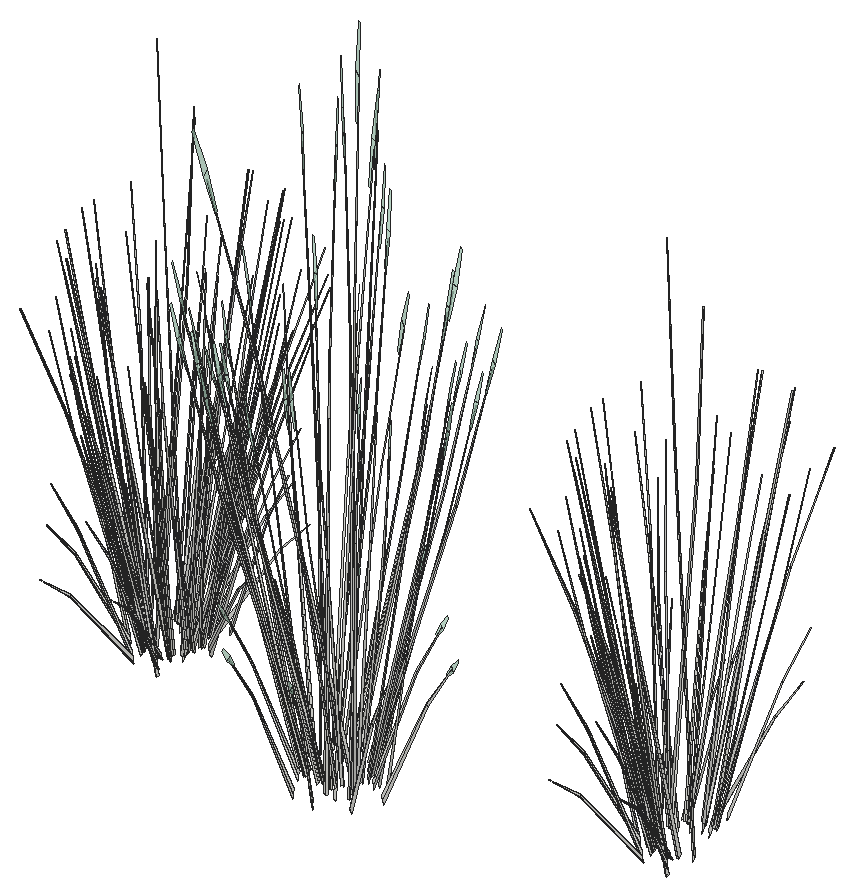
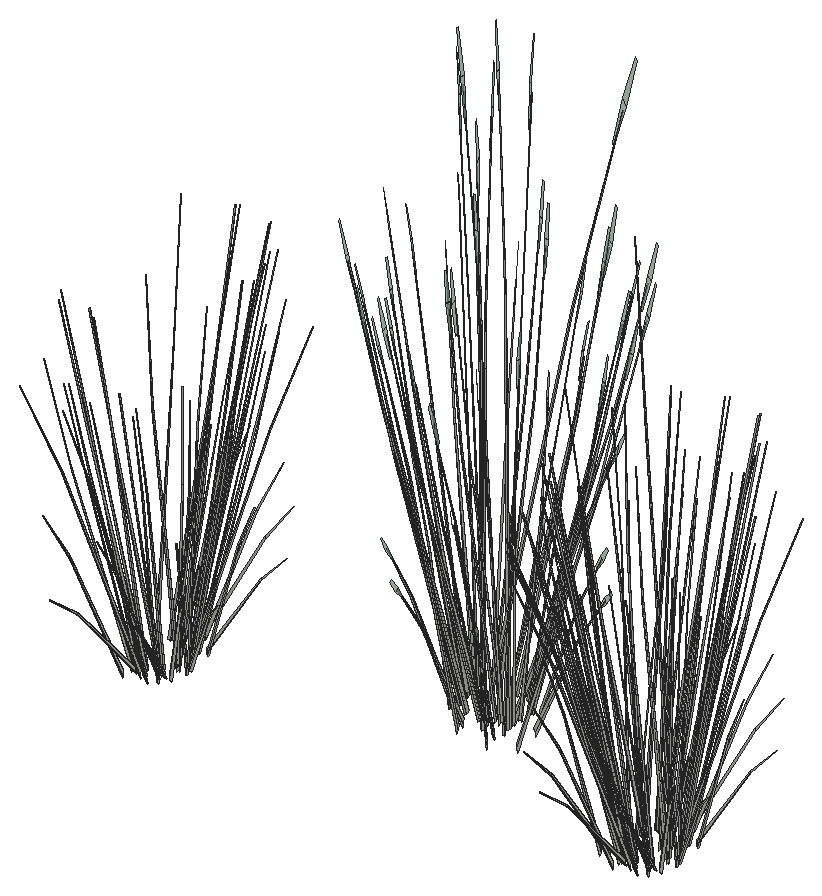
# SketchUp Ruby script. Lengths in inches.
U = 1.inch
M = Sketchup.active_model
def pt(a) = Geom::Point3d.new(a.map { |v| v * U })
def face(e, loops, mat)
  f = e.add_face(loops[0].map { |a| pt(a) })
  loops[1..].each { |l| e.add_face(l.map { |a| pt(a) }).erase! }
  f.material = f.back_material = mat if mat
  f
end
# faces: each face lists its corners as indices into pts; further lists are holes
def faces(e, pts, list, mat = nil) = list.each { |f| face(e, (f[0].is_a?(Array) ? f : [f]).map { |l| l.map { |i| pts[i] } }, mat) }
# xy, xz, yz: faces in a plane at the given z, y or x. An outline is a flat list of corners, or four numbers for a rectangle; further outlines are holes
def ring(l) = l.size == 4 ? [[l[0], l[1]], [l[2], l[1]], [l[2], l[3]], [l[0], l[3]]] : l.each_slice(2).to_a
def flat(e, list, mat, &to3) = list.each { |f| face(e, (f[0].is_a?(Array) ? f : [f]).map { |l| ring(l).map { |u, v| to3.(u, v) } }, mat) }
def xy(e, z, list, mat = nil) = flat(e, list, mat) { |x, y| [x, y, z] }
def xz(e, y, list, mat = nil) = flat(e, list, mat) { |x, z| [x, y, z] }
def yz(e, x, list, mat = nil) = flat(e, list, mat) { |y, z| [x, y, z] }
def lines(e, pts, list) = list.each { |a, b| e.add_line(pt(pts[a]), pt(pts[b])) }
# prism: a flat outline (further loops are holes) pulled along v
def prism(e, loops, v, mat = nil)
  f = face(e, loops, mat); d = Geom::Vector3d.new(v.map { |x| x * U })
  f.pushpull(f.normal.samedirection?(d) ? d.length : -d.length)
end
def box(e, o, s, mat = nil) = prism(e, [[o, [o[0] + s[0], o[1], o[2]], [o[0] + s[0], o[1] + s[1], o[2]], [o[0], o[1] + s[1], o[2]]]], [0, 0, s[2]], mat)
def at(x, y, z, deg = 0) = Geom::Transformation.translation(pt([x, y, z])) * Geom::Transformation.rotation(ORIGIN, Z_AXIS, deg.degrees)
def axes(o, x, y, z) = Geom::Transformation.new([*x, 0, *y, 0, *z, 0, *pt(o).to_a, 1])
def part(name) = M.definitions.add(name)
# library, detail: a bought-in or finely detailed component or shape, given as its bounding box
def library(name, o, s) = part(name).tap { |d| box(d.entities, o, s) }
def detail(e, o, s) = box(e.add_group.entities, o, s)
def put(e, d, t, mat = nil) = e.add_instance(d, t).tap { |i| i.material = mat if mat }
def group(e, t, mat = nil) = e.add_group.tap { |g| g.transformation = t; g.material = mat if mat }.entities
root = M.entities
M.materials.add("LightPink_Translucent").color = [175, 214, 192]
M.materials["LightPink_Translucent"].alpha = 0.75
c1 = part("blade")
p = [[2.15,0.21,22],[0,0.17,0],[0.09,0.45,0],[2.18,0.31,22],[2.29,0.31,22],[0.38,0.45,0],
  [2.48,0.24,33],[2.49,0.24,33],[2.48,0.22,33]]
faces(c1.entities,p,[[0,1,2,3],[4,5,2,3],[6,3,4,7],[8,0,3,6]])
c2 = part("blade with seeds\#1")
put(c2.entities,c1,at(0,0,0))
c3 = part("seeds")
p = [[0.3,-0.1,1.38],[-0.01,-0.03,1.59],[-0.01,-0.03,0.03],[0.14,-0.07,-0.07],[0.29,-0.03,3],[0.15,0.01,3.11]]
faces(c3.entities,p,[[0,1,2,3],[1,0,4,5]],"LightPink_Translucent")
c4 = part("blade with seeds")
put(c4.entities,c1,at(0,0,0))
put(c4.entities,c3,axes([2.4,0.25,30.99],[1.5799,-0.05474,1.17369],[-0.12525,1.92788,0.29478],[-0.07173,-0.02425,1.56792]))
put(root,c2,axes([371.53,244.35,139.9],[0.12234,-0.11364,1.40588],[0.103,0.52511,0.11368],[-0.19206,0.11868,0.601]))
put(root,c2,axes([370.72,243.48,140.59],[-0.05342,0.07604,1.43516],[0.03387,0.50744,-0.22697],[-0.12778,0.08099,0.1151]))
put(root,c2,axes([371.1,241.31,140.58],[0.0291,0.05049,1.45516],[-0.09819,0.49465,-0.1375],[-0.12701,0.01791,0.25751]))
put(root,c2,axes([371.375,241.2,140.59],[-0.07584,0.0048,1.43516],[-0.21918,0.40531,-0.22697],[-0.13286,-0.06266,0.1151]))
put(root,c2,axes([371.75,242.57,139.9],[0.13097,0.09256,1.40588],[-0.27104,0.38832,0.11368],[-0.16893,-0.17518,0.601]))
put(root,c2,axes([371.36,242.9,140.43],[-0.29303,-0.14987,-0.29052],[0.08547,-0.43725,0.37506],[-0.11798,0.04009,0.71765]))
put(root,c2,axes([370.54,244,140.58],[0.04567,0.00927,1.45516],[0.16576,0.45742,-0.1375],[-0.08473,0.1346,0.25751]))
put(root,c2,axes([371.54,242.71,140.85],[0.17741,0.48648,-0.09976],[-0.31487,0.23906,-0.55369],[-0.13269,0.06419,0.84132]))
put(root,c2,axes([371.43,242.85,140.6],[0.09962,-0.48986,0.39379],[0.3275,0.16751,0.3247],[-0.12879,0.02944,0.81485]))
put(root,c2,axes([371.94,241.7,140.85],[-0.01888,0.54637,-0.09976],[-0.35746,-0.01493,-0.55369],[-0.13767,-0.03795,0.84132]))
put(root,c2,axes([371.4,242.72,140.6],[-0.1295,-0.36632,0.05275],[0.23615,-0.1793,0.41527],[-0.1041,0.03538,0.63322]))
put(root,c2,axes([371.47,244.16,140.43],[-0.30692,0.07678,-0.29052],[-0.08104,-0.43892,0.37506],[-0.08795,0.11789,0.71765]))
put(root,c2,axes([371.71,241.73,140.43],[-0.20062,-0.33637,-0.29052],[0.22908,-0.31842,0.37506],[-0.11639,-0.04845,0.71765]))
put(root,c2,axes([371.4375,243.97,140.6],[-0.24206,-0.22594,0.05275],[0.14093,-0.32175,0.41527],[-0.07761,0.10402,0.63322]))
put(root,c2,axes([371.91,245.11,139.9],[0.06565,-0.18466,1.40588],[0.27542,0.38215,0.11368],[-0.12424,0.23818,0.601]))
put(root,c2,axes([371.41,243.87,141.17],[0.3653,0.33178,-0.11173],[-0.21045,0.48049,-0.62013],[-0.10321,0.16702,0.94228]))
put(root,c2,axes([371.79,241.74,140.6],[0.25999,-0.354,0.39379],[0.22422,0.37594,0.3247],[-0.12198,-0.0653,0.81485]))
put(root,c2,axes([371.81,241.61,140.6],[0.01775,-0.40853,0.05275],[0.2681,0.0112,0.41527],[-0.1027,-0.04275,0.63322]))
put(root,c2,axes([371.31,245.14,140.59],[-0.00269,0.10696,1.43516],[0.26896,0.34054,-0.22697],[-0.05496,0.1817,0.1151]))
put(root,c2,axes([372.65,241.1,140.85],[-0.21011,0.45986,-0.09976],[-0.30427,-0.26493,-0.55369],[-0.10577,-0.12992,0.84132]))
put(root,c2,axes([372.55,239.97,140.58],[-0.00289,0.06493,1.45516],[-0.31009,0.26964,-0.1375],[-0.10196,-0.10828,0.25751]))
put(root,c2,axes([373.79,243,139.45],[0.15365,-0.4296,1.24087],[0.33102,0.42086,0.4907],[-0.19619,0.18851,1.04025]))
put(root,c2,axes([371.91,245.03,140.6],[-0.28975,-0.02503,0.05275],[0.00794,-0.378,0.41527],[-0.03032,0.1448,0.63322]))
put(root,c2,axes([372.01,245.18,140.43],[-0.23857,0.28286,-0.29052],[-0.22584,-0.32298,0.37506],[-0.03436,0.1641,0.71765]))
put(root,c2,axes([372.43,240.97,140.43],[-0.05446,-0.43273,-0.29052],[0.31131,-0.11427,0.37506],[-0.08362,-0.12401,0.71765]))
put(root,c2,axes([372.5,241.03,140.6],[0.35069,-0.12329,0.39379],[0.06086,0.48364,0.3247],[-0.08248,-0.14254,0.81485]))
put(root,c2,axes([372.57,240.93,140.6],[0.16025,-0.34128,0.05275],[0.22821,0.1987,0.41527],[-0.07378,-0.10942,0.63322]))
put(root,c2,axes([372.92,239.73,140.59],[-0.05804,-0.06898,1.43516],[-0.35603,0.0883,-0.22697],[-0.0675,-0.17309,0.1151]))
put(root,c2,axes([371.53,245.55,140.58],[0.03803,-0.03685,1.45516],[0.34183,0.17767,-0.1375],[0.00247,0.17994,0.25751]))
put(root,c2,axes([371.98,244.86,140.85],[0.38751,0.02662,-0.09976],[-0.01059,0.50399,-0.55369],[-0.02692,0.19411,0.84132]))
put(root,c2,axes([373.47,241.08,140.85],[-0.34504,0.25013,-0.09976],[-0.16956,-0.44394,-0.55369],[-0.04552,-0.18708,0.84132]))
put(root,c2,axes([372.51,245.5,139.9],[-0.00863,-0.2062,1.40588],[0.37404,0.13679,0.11368],[-0.02314,0.29386,0.601]))
put(root,c2,axes([372.79,245.58,140.6],[-0.34743,-0.14045,0.39379],[0.1188,-0.46175,0.3247],[0.02088,0.18159,0.81485]))
put(root,c2,axes([372.7,245.62,140.6],[-0.25981,0.18259,0.05275],[-0.12717,-0.33295,0.41527],[0.02509,0.14677,0.63322]))
put(root,c2,axes([372.83,245.68,140.43],[-0.1063,0.41315,-0.29052],[-0.31012,-0.1205,0.37506],[0.02844,0.16634,0.71765]))
put(root,c2,axes([373.33,240.82,140.43],[0.1063,-0.41315,-0.29052],[0.31012,0.1205,0.37506],[-0.02844,-0.16634,0.71765]))
put(root,c2,axes([372.94,241.95,139.9],[0.00863,0.2062,1.40588],[-0.37404,-0.13679,0.11368],[0.02314,-0.29386,0.601]))
put(root,c2,axes([373.46,240.88,140.6],[0.25981,-0.18259,0.05275],[0.12717,0.33295,0.41527],[-0.02509,-0.14677,0.63322]))
put(root,c2,axes([373.37,240.92,140.6],[0.34743,0.14045,0.39379],[-0.1188,0.46175,0.3247],[-0.02088,-0.18159,0.81485]))
put(root,c2,axes([372.69,245.42,140.85],[0.34504,-0.25013,-0.09976],[0.16956,0.44394,-0.55369],[0.04552,0.18708,0.84132]))
put(root,c2,axes([374.49,240.09,140.58],[-0.03336,0.04495,1.45516],[-0.35758,-0.09833,-0.1375],[-0.02285,-0.17707,0.25751]))
put(root,c2,axes([373.04,245.9375,140.59],[0.04947,0.08118,1.43516],[0.36146,-0.00691,-0.22697],[0.04701,0.18608,0.1151]))
put(root,c2,axes([374.19,240.48,139.94],[-0.32031,0.09515,-0.02864],[-0.07364,-0.44972,-0.12987],[0.02031,-0.09391,0.42837]))
put(root,c2,axes([374.18,241.65,140.85],[-0.38751,-0.02662,-0.09976],[0.01059,-0.50399,-0.55369],[0.02692,-0.19411,0.84132]))
put(root,c2,axes([373.95,241.21,140.59],[-0.00644,-0.10664,1.43516],[-0.29603,-0.29251,-0.22697],[0.03908,-0.18969,0.1151]))
put(root,c2,axes([373.59,245.57,140.6],[-0.16025,0.34128,0.05275],[-0.22821,-0.1987,0.41527],[0.07378,0.10942,0.63322]))
put(root,c2,axes([373.66,245.47,140.6],[-0.35069,0.12329,0.39379],[-0.06086,-0.48364,0.3247],[0.08248,0.14254,0.81485]))
put(root,c2,axes([373.17,245.41,139.9],[-0.0806,-0.17249,1.40588],[0.37244,-0.14522,0.11368],[0.08417,0.2708,0.601]))
put(root,c2,axes([373.4,246.84,140.58],[0.01022,-0.06344,1.45516],[0.33667,-0.19627,-0.1375],[0.08837,0.12987,0.25751]))
put(root,c2,axes([373.73,245.53,140.43],[0.05446,0.43273,-0.29052],[-0.31131,0.11427,0.37506],[0.08362,0.12401,0.71765]))
put(root,c2,axes([374.16,241.32,140.43],[0.23857,-0.28286,-0.29052],[0.22584,0.32298,0.37506],[0.03436,-0.1641,0.71765]))
put(root,c2,axes([374.25,241.47,140.6],[0.28975,0.02503,0.05275],[-0.00794,0.378,0.41527],[0.03032,-0.1448,0.63322]))
put(root,c2,axes([374.15,241.43,140.6],[0.25108,0.36656,0.39379],[-0.26664,0.31614,0.3247],[0.04631,-0.17198,0.81485]))
put(root,c2,axes([372.68,242.3,140.39],[-0.19798,0.42958,1.1344],[-0.30825,-0.45359,0.48946],[0.18577,-0.1386,1.09651]))
put(root,c2,axes([373.54,242.34,139.9],[-0.06565,0.18466,1.40588],[-0.27542,-0.38215,0.11368],[0.12424,-0.23818,0.601]))
put(root,c2,axes([373.51,245.4,140.85],[0.21011,-0.45986,-0.09976],[0.30427,0.26493,-0.55369],[0.10577,0.12992,0.84132]))
put(root,c2,axes([373.42,244.78,139.9],[-0.11708,-0.12417,1.40588],[0.31602,-0.31352,0.11368],[0.14392,0.21504,0.601]))
put(root,c2,axes([374.6,242.64,140.85],[-0.32616,-0.29624,-0.09976],[0.1879,-0.42901,-0.55369],[0.09215,-0.14913,0.84132]))
put(root,c2,axes([374.35,244.89,140.6],[-0.01775,0.40853,0.05275],[-0.2681,-0.0112,0.41527],[0.1027,0.04275,0.63322]))
put(root,c2,axes([374.875,243.02,140.58],[-0.04613,-0.00147,1.45516],[-0.20353,-0.42603,-0.1375],[0.07265,-0.14798,0.25751]))
put(root,c2,axes([374.37,244.76,140.6],[-0.25999,0.354,0.39379],[-0.22422,-0.37594,0.3247],[0.12198,0.0653,0.81485]))
put(root,c2,axes([374.72,242.53,140.6],[0.24206,0.22594,0.05275],[-0.14093,0.32175,0.41527],[0.07761,-0.10402,0.63322]))
put(root,c2,axes([374.66,242.43,140.6],[0.08745,0.49445,0.39379],[-0.34303,0.08581,0.3247],[0.1011,-0.11629,0.81485]))
put(root,c2,axes([373.71,244.87,139.9],[-0.13097,-0.09256,1.40588],[0.27104,-0.38832,0.11368],[0.16893,0.17518,0.601]))
put(root,c2,axes([374.45,244.77,140.43],[0.20062,0.33637,-0.29052],[-0.22908,0.31842,0.37506],[0.11639,0.04845,0.71765]))
put(root,c2,axes([374.76,243.78,140.6],[0.1295,0.36632,0.05275],[-0.23615,0.1793,0.41527],[0.1041,-0.03538,0.63322]))
put(root,c2,axes([374.39,245.93,140.59],[0.0754,0.01236,1.43516],[0.26232,-0.35069,-0.22697],[0.12405,0.09181,0.1151]))
put(root,c2,axes([374.22,244.8,141.15],[0.01888,-0.54637,-0.11073],[0.35746,0.01493,-0.6146],[0.13767,0.03795,0.93387]))
put(root,c2,axes([374.62,243.79,140.85],[-0.17741,-0.48648,-0.09976],[0.31487,-0.23906,-0.55369],[0.13269,-0.06419,0.84132]))
put(root,c2,axes([373.93,243.1,139.9],[-0.12234,0.11364,1.40588],[-0.103,-0.52511,0.11368],[0.19206,-0.11868,0.601]))
put(root,c2,axes([374.8,243.6,140.43],[0.29303,0.14987,-0.29052],[-0.08547,0.43725,0.37506],[0.11798,-0.04009,0.71765]))
put(root,c2,axes([373.99,244.03,139.9],[-0.14625,0.01217,1.40588],[0.09702,-0.52737,0.11368],[0.20842,0.03262,0.601]))
put(root,c2,axes([375.16,245.97,140.58],[-0.02301,-0.0564,1.45516],[0.15302,-0.46615,-0.1375],[0.12741,0.01095,0.25751]))
put(root,c2,axes([375.32,243.91,140.59],[0.06136,-0.06302,1.43516],[0.02411,-0.50855,-0.22697],[0.13532,-0.05114,0.1151]))
put(root,c2,axes([374.73,244.72,139.48],[-0.19671,-0.01092,1.26617],[0.1039,-0.49126,0.17497],[0.20964,0.04257,0.59789]))
put(root,c4,axes([389.69,236,140.21],[0.13585,-0.06442,1.61128],[0.04685,0.4498,0.1261],[-0.29426,0.05969,0.57588]))
put(root,c4,axes([389.25,235.28,141.7],[-0.47777,-0.01072,-0.64651],[0.03209,-0.45152,0.07802],[-0.2024,-0.04765,0.91455]))
put(root,c4,axes([388.48,236.0625,141.29],[-0.3972,-0.12423,-0.32227],[0.11585,-0.36244,0.41605],[-0.15992,0.03323,0.79608]))
put(root,c4,axes([388.75,236.25,141.43],[-0.12948,0.40508,-0.465],[-0.44393,-0.13885,-0.36018],[-0.17873,0.03714,0.88973]))
put(root,c4,axes([389.09,235.375,141.43],[-0.34704,0.29499,-0.465],[-0.30393,-0.31162,-0.36018],[-0.17633,-0.04488,0.88973]))
put(root,c4,axes([387.875,237.98,139.6875],[0.19918,-0.20183,1.04523],[0.0786,0.31952,0.76796],[-0.14394,0.05721,0.23022]))
put(root,c4,axes([388.96,235.1,141.29],[-0.27194,-0.27882,-0.32227],[0.31051,-0.26394,0.41605],[-0.15777,-0.04016,0.79608]))
put(root,c4,axes([388.625,237.11,141.29],[-0.41603,0.06364,-0.32227],[-0.10985,-0.36383,0.41605],[-0.11922,0.09772,0.79608]))
put(root,c4,axes([388.31,235.76,139.6875],[0.30513,-0.03187,1.04523],[-0.19355,0.28077,0.76796],[-0.15079,-0.04212,0.23022]))
put(root,c4,axes([388.97,237.15,141.43],[0.12278,0.40663,-0.465],[-0.46497,0.07113,-0.36018],[-0.13325,0.10922,0.88973]))
put(root,c4,axes([390.08,234.75,141.7],[-0.40754,-0.21525,-0.64651],[0.28963,-0.37719,0.07802],[-0.14765,-0.12852,0.91455]))
put(root,c4,axes([389.89,234.76,141.43],[-0.47162,0.10586,-0.465],[-0.0825,-0.4009,-0.36018],[-0.12667,-0.11489,0.88973]))
put(root,c4,axes([389.9375,234.47,141.29],[-0.07382,-0.3587,-0.32227],[0.42197,-0.09472,0.41605],[-0.11334,-0.10279,0.79608]))
put(root,c4,axes([389.36,237.95,141.29],[-0.32338,0.23447,-0.32227],[-0.30612,-0.26773,0.41605],[-0.04658,0.13603,0.79608]))
put(root,c4,axes([391.05,237.19,140.2],[0.41302,0.17958,1.37647],[-0.40462,0.38687,0.54432],[-0.18124,-0.22929,1.15394]))
put(root,c4,axes([389.48,233.93,139.6875],[0.24931,0.155,1.04523],[-0.36309,0.09317,0.76796],[-0.07769,-0.11912,0.23022]))
put(root,c4,axes([389.57,237.7,142.03],[-0.01244,0.41193,-0.71763],[-0.52368,-0.02767,0.0866],[-0.05527,0.17451,1.01516]))
put(root,c4,axes([389.56,238.86,139.6875],[-0.01237,-0.2648,1.04523],[0.30908,0.18886,0.76796],[-0.06079,0.12621,0.23022]))
put(root,c4,axes([389.4,238.28,140.23],[0.0105,-0.22989,1.40454],[0.4723,0.12143,0.19409],[-0.04092,0.24501,0.66323]))
put(root,c4,axes([389.68,237.84,141.72],[0.34214,0.29922,-0.51615],[-0.36143,0.26205,-0.3998],[-0.05206,0.15203,0.9876]))
put(root,c4,axes([391.7,236.33,139.76],[-0.01306,-0.4193,1.28558],[0.59089,0.10869,0.54432],[-0.13975,0.22943,1.21348]))
put(root,c4,axes([390.9375,234.57,141.43],[-0.46982,-0.11164,-0.465],[0.16104,-0.38276,-0.36018],[-0.04308,-0.1541,0.88973]))
put(root,c4,axes([390.34,236.58,139.64],[-0.23189,0.40128,0.40713],[-0.48183,-0.19312,-0.19594],[0,-0.0925,1.30716]))
put(root,c4,axes([391.11,234.65,141.7],[-0.22811,-0.3621,-0.64651],[0.46957,-0.2018,0.07802],[-0.05334,-0.17496,0.91455]))
put(root,c4,axes([391.46,236.76,139.64],[0.519,-0.02749,0.40713],[0.04694,0.45634,-0.19594],[-0.09291,0.04625,1.30716]))
put(root,c4,axes([391.15,234.34,141.29],[0.14409,-0.34247,-0.32227],[0.42037,0.09989,0.41605],[-0.03855,-0.13788,0.79608]))
put(root,c4,axes([390.48,238.37,141.29],[-0.14409,0.34247,-0.32227],[-0.42037,-0.09989,0.41605],[0.03855,0.13788,0.79608]))
put(root,c4,axes([390.46,236.02,139.64],[-0.519,0.02749,0.40713],[-0.04694,-0.45634,-0.19594],[0.09291,-0.04625,1.30716]))
put(root,c4,axes([390.52,238.06,141.7],[0.22811,0.3621,-0.64651],[-0.46957,0.2018,0.07802],[0.05334,0.17496,0.91455]))
put(root,c4,axes([391.23,233.62,139.6875],[0.06131,0.25968,1.04523],[-0.34012,-0.14383,0.76796],[0.0366,-0.13297,0.23022]))
put(root,c4,axes([391.58,236.21,139.64],[0.23189,-0.40128,0.40713],[0.48183,0.19312,-0.19594],[0,0.0925,1.30716]))
put(root,c4,axes([390.7,238.13,141.43],[0.46982,0.11164,-0.465],[-0.16104,0.38276,-0.36018],[0.04308,0.1541,0.88973]))
put(root,c4,axes([391.08,235.84,139.64],[-0.28711,-0.37379,0.40713],[0.43489,-0.26322,-0.19594],[0.09291,0.04625,1.30716]))
put(root,c4,axes([391.95,234.86,141.43],[-0.34214,-0.29922,-0.465],[0.36143,-0.26205,-0.36018],[0.05206,-0.15203,0.88973]))
put(root,c4,axes([392.06,235,141.7],[0.01244,-0.41193,-0.64651],[0.52368,0.02767,0.07802],[0.05527,-0.17451,0.91455]))
put(root,c4,axes([392.27,234.75,141.29],[0.32338,-0.23447,-0.32227],[0.30612,0.26773,0.41605],[0.04658,-0.13603,0.79608]))
put(root,c4,axes([392.35,237.77,139.6875],[-0.2691,-0.12805,1.04523],[0.34747,-0.13011,0.76796],[0.09372,0.11021,0.23022]))
put(root,c4,axes([392.39,238.35,139.6],[-0.30649,-0.01397,0.95605],[0.2024,-0.29664,0.52785],[0.12108,0.10539,0.74993]))
put(root,c4,axes([391.74,237.94,141.43],[0.47162,-0.10586,-0.465],[0.0825,0.4009,-0.36018],[0.12667,0.11489,0.88973]))
put(root,c4,axes([392.66,235.55,141.43],[-0.12278,-0.40663,-0.465],[0.46497,-0.07113,-0.36018],[0.13325,-0.10922,0.88973]))
put(root,c4,axes([393.48,237.65,140.75],[-0.09148,-0.37435,-0.03177],[0.43236,-0.08606,-0.14407],[0.09029,0.02373,0.47519]))
put(root,c4,axes([393.23,234.74,139.6875],[-0.15919,0.2267,1.04523],[-0.13683,-0.30457,0.76796],[0.13148,-0.07632,0.23022]))
put(root,c4,axes([393,235.6,141.29],[0.41603,-0.06364,-0.32227],[0.10985,0.36383,0.41605],[0.11922,-0.09772,0.79608]))
put(root,c4,axes([392.67,235.72,141.7],[0.24965,-0.35138,-0.64651],[0.43748,0.24972,0.07802],[0.14906,-0.12731,0.91455]))
put(root,c4,axes([392.67,237.61,141.29],[0.27194,0.27882,-0.32227],[-0.31051,0.26394,0.41605],[0.15777,0.04016,0.79608]))
put(root,c4,axes([392.88,236.46,141.43],[0.12948,-0.40508,-0.465],[0.44393,0.13885,-0.36018],[0.17873,-0.03714,0.88973]))
put(root,c4,axes([393.99,236.71,139.6875],[-0.2953,0.07352,1.04523],[0.139,-0.30384,0.76796],[0.15666,0.02079,0.23022]))
put(root,c4,axes([393.15,236.64,141.29],[0.3972,0.12423,-0.32227],[-0.11585,0.36244,0.41605],[0.15992,-0.03323,0.79608]))
put(root,c4,axes([392.38,237.42,141.7],[0.47777,0.01072,-0.64651],[-0.03209,0.45152,0.07802],[0.2024,0.04765,0.91455]))
put(root,c4,axes([392.79,236.6,141.7],[0.41997,-0.19668,-0.64651],[0.23405,0.40486,0.07802],[0.20292,-0.04599,0.91455]))
put(root,c2,axes([409.72,244.35,139.9],[0.12234,-0.11364,1.40588],[0.103,0.52511,0.11368],[-0.19206,0.11868,0.601]))
put(root,c2,axes([408.91,243.48,140.59],[-0.05342,0.07604,1.43516],[0.03387,0.50744,-0.22697],[-0.12778,0.08099,0.1151]))
put(root,c2,axes([409.3,241.31,140.58],[0.0291,0.05049,1.45516],[-0.09819,0.49465,-0.1375],[-0.12701,0.01791,0.25751]))
put(root,c2,axes([409.57,241.2,140.59],[-0.07584,0.0048,1.43516],[-0.21918,0.40531,-0.22697],[-0.13286,-0.06266,0.1151]))
put(root,c2,axes([409.94,242.57,139.9],[0.13097,0.09256,1.40588],[-0.27104,0.38832,0.11368],[-0.16893,-0.17518,0.601]))
put(root,c2,axes([409.55,242.9,140.43],[-0.29303,-0.14987,-0.29052],[0.08547,-0.43725,0.37506],[-0.11798,0.04009,0.71765]))
put(root,c2,axes([408.74,244,140.58],[0.04567,0.00927,1.45516],[0.16576,0.45742,-0.1375],[-0.08473,0.1346,0.25751]))
put(root,c2,axes([409.74,242.71,140.85],[0.17741,0.48648,-0.09976],[-0.31487,0.23906,-0.55369],[-0.13269,0.06419,0.84132]))
put(root,c2,axes([409.62,242.85,140.6],[0.09962,-0.48986,0.39379],[0.3275,0.16751,0.3247],[-0.12879,0.02944,0.81485]))
put(root,c2,axes([410.14,241.7,140.85],[-0.01888,0.54637,-0.09976],[-0.35746,-0.01493,-0.55369],[-0.13767,-0.03795,0.84132]))
put(root,c2,axes([409.6,242.72,140.6],[-0.1295,-0.36632,0.05275],[0.23615,-0.1793,0.41527],[-0.1041,0.03538,0.63322]))
put(root,c2,axes([409.66,244.16,140.43],[-0.30692,0.07678,-0.29052],[-0.08104,-0.43892,0.37506],[-0.08795,0.11789,0.71765]))
put(root,c2,axes([409.91,241.73,140.43],[-0.20062,-0.33637,-0.29052],[0.22908,-0.31842,0.37506],[-0.11639,-0.04845,0.71765]))
put(root,c2,axes([409.63,243.97,140.6],[-0.24206,-0.22594,0.05275],[0.14093,-0.32175,0.41527],[-0.07761,0.10402,0.63322]))
put(root,c2,axes([410.11,245.11,139.9],[0.06565,-0.18466,1.40588],[0.27542,0.38215,0.11368],[-0.12424,0.23818,0.601]))
put(root,c2,axes([409.61,243.87,141.17],[0.3653,0.33178,-0.11173],[-0.21045,0.48049,-0.62013],[-0.10321,0.16702,0.94228]))
put(root,c2,axes([409.98,241.74,140.6],[0.25999,-0.354,0.39379],[0.22422,0.37594,0.3247],[-0.12198,-0.0653,0.81485]))
put(root,c2,axes([410.01,241.61,140.6],[0.01775,-0.40853,0.05275],[0.2681,0.0112,0.41527],[-0.1027,-0.04275,0.63322]))
put(root,c2,axes([409.5,245.14,140.59],[-0.00269,0.10696,1.43516],[0.26896,0.34054,-0.22697],[-0.05496,0.1817,0.1151]))
put(root,c2,axes([410.84,241.1,140.85],[-0.21011,0.45986,-0.09976],[-0.30427,-0.26493,-0.55369],[-0.10577,-0.12992,0.84132]))
put(root,c2,axes([410.75,239.97,140.58],[-0.00289,0.06493,1.45516],[-0.31009,0.26964,-0.1375],[-0.10196,-0.10828,0.25751]))
put(root,c2,axes([411.99,243,139.45],[0.15365,-0.4296,1.24087],[0.33102,0.42086,0.4907],[-0.19619,0.18851,1.04025]))
put(root,c2,axes([410.11,245.03,140.6],[-0.28975,-0.02503,0.05275],[0.00794,-0.378,0.41527],[-0.03032,0.1448,0.63322]))
put(root,c2,axes([410.2,245.18,140.43],[-0.23857,0.28286,-0.29052],[-0.22584,-0.32298,0.37506],[-0.03436,0.1641,0.71765]))
put(root,c2,axes([410.63,240.97,140.43],[-0.05446,-0.43273,-0.29052],[0.31131,-0.11427,0.37506],[-0.08362,-0.12401,0.71765]))
put(root,c2,axes([410.69,241.03,140.6],[0.35069,-0.12329,0.39379],[0.06086,0.48364,0.3247],[-0.08248,-0.14254,0.81485]))
put(root,c2,axes([410.76,240.93,140.6],[0.16025,-0.34128,0.05275],[0.22821,0.1987,0.41527],[-0.07378,-0.10942,0.63322]))
put(root,c2,axes([411.12,239.73,140.59],[-0.05804,-0.06898,1.43516],[-0.35603,0.0883,-0.22697],[-0.0675,-0.17309,0.1151]))
put(root,c2,axes([409.73,245.55,140.58],[0.03803,-0.03685,1.45516],[0.34183,0.17767,-0.1375],[0.00247,0.17994,0.25751]))
put(root,c2,axes([410.17,244.86,140.85],[0.38751,0.02662,-0.09976],[-0.01059,0.50399,-0.55369],[-0.02692,0.19411,0.84132]))
put(root,c2,axes([411.66,241.08,140.85],[-0.34504,0.25013,-0.09976],[-0.16956,-0.44394,-0.55369],[-0.04552,-0.18708,0.84132]))
put(root,c2,axes([410.71,245.5,139.9],[-0.00863,-0.2062,1.40588],[0.37404,0.13679,0.11368],[-0.02314,0.29386,0.601]))
put(root,c2,axes([410.99,245.58,140.6],[-0.34743,-0.14045,0.39379],[0.1188,-0.46175,0.3247],[0.02088,0.18159,0.81485]))
put(root,c2,axes([410.9,245.62,140.6],[-0.25981,0.18259,0.05275],[-0.12717,-0.33295,0.41527],[0.02509,0.14677,0.63322]))
put(root,c2,axes([411.03,245.68,140.43],[-0.1063,0.41315,-0.29052],[-0.31012,-0.1205,0.37506],[0.02844,0.16634,0.71765]))
put(root,c2,axes([411.52,240.82,140.43],[0.1063,-0.41315,-0.29052],[0.31012,0.1205,0.37506],[-0.02844,-0.16634,0.71765]))
put(root,c2,axes([411.14,241.95,139.9],[0.00863,0.2062,1.40588],[-0.37404,-0.13679,0.11368],[0.02314,-0.29386,0.601]))
put(root,c2,axes([411.65,240.88,140.6],[0.25981,-0.18259,0.05275],[0.12717,0.33295,0.41527],[-0.02509,-0.14677,0.63322]))
put(root,c2,axes([411.56,240.92,140.6],[0.34743,0.14045,0.39379],[-0.1188,0.46175,0.3247],[-0.02088,-0.18159,0.81485]))
put(root,c2,axes([410.89,245.42,140.85],[0.34504,-0.25013,-0.09976],[0.16956,0.44394,-0.55369],[0.04552,0.18708,0.84132]))
put(root,c2,axes([412.68,240.09,140.58],[-0.03336,0.04495,1.45516],[-0.35758,-0.09833,-0.1375],[-0.02285,-0.17707,0.25751]))
put(root,c2,axes([411.23,245.9375,140.59],[0.04947,0.08118,1.43516],[0.36146,-0.00691,-0.22697],[0.04701,0.18608,0.1151]))
put(root,c2,axes([412.39,240.48,139.94],[-0.32031,0.09515,-0.02864],[-0.07364,-0.44972,-0.12987],[0.02031,-0.09391,0.42837]))
put(root,c2,axes([412.375,241.65,140.85],[-0.38751,-0.02662,-0.09976],[0.01059,-0.50399,-0.55369],[0.02692,-0.19411,0.84132]))
put(root,c2,axes([412.14,241.21,140.59],[-0.00644,-0.10664,1.43516],[-0.29603,-0.29251,-0.22697],[0.03908,-0.18969,0.1151]))
put(root,c2,axes([411.79,245.57,140.6],[-0.16025,0.34128,0.05275],[-0.22821,-0.1987,0.41527],[0.07378,0.10942,0.63322]))
put(root,c2,axes([411.85,245.47,140.6],[-0.35069,0.12329,0.39379],[-0.06086,-0.48364,0.3247],[0.08248,0.14254,0.81485]))
put(root,c2,axes([411.36,245.41,139.9],[-0.0806,-0.17249,1.40588],[0.37244,-0.14522,0.11368],[0.08417,0.2708,0.601]))
put(root,c2,axes([411.6,246.84,140.58],[0.01022,-0.06344,1.45516],[0.33667,-0.19627,-0.1375],[0.08837,0.12987,0.25751]))
put(root,c2,axes([411.92,245.53,140.43],[0.05446,0.43273,-0.29052],[-0.31131,0.11427,0.37506],[0.08362,0.12401,0.71765]))
